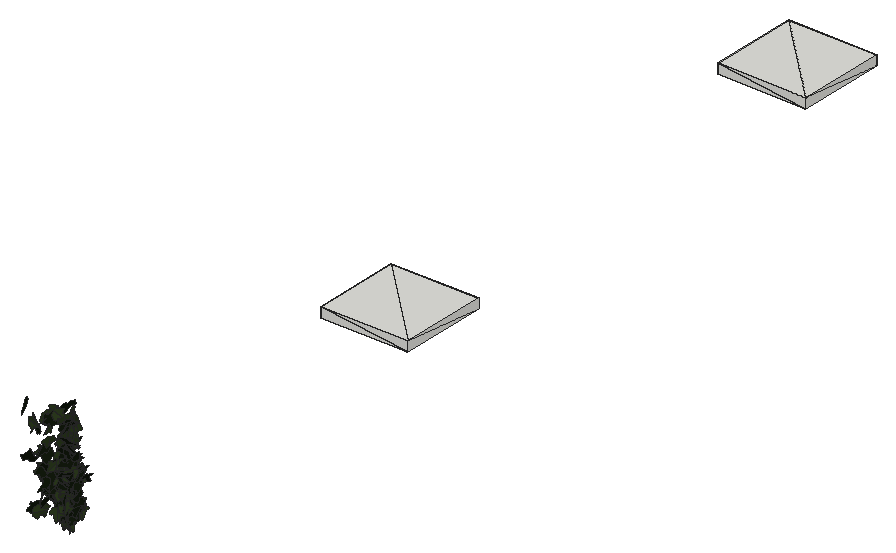
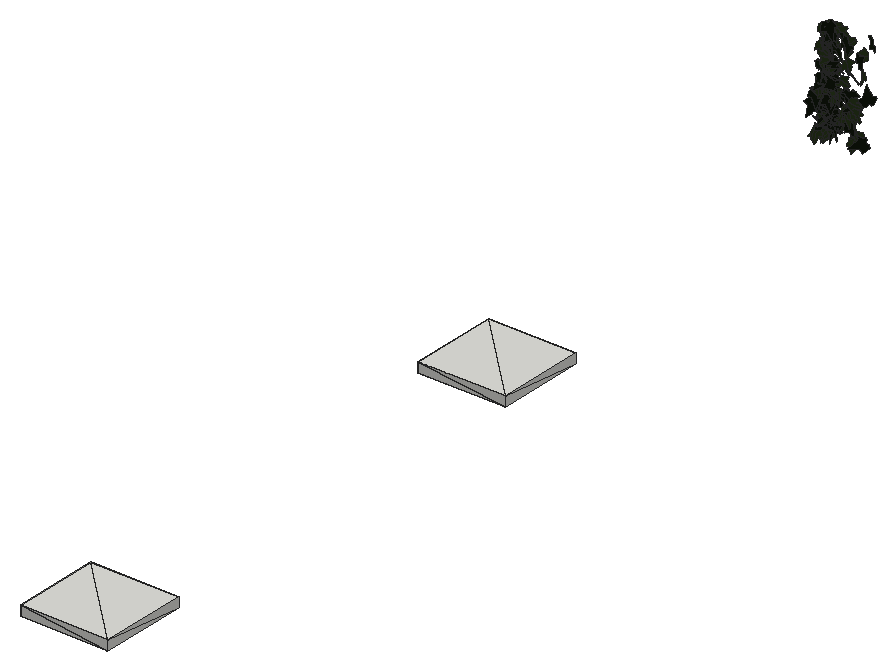
# SketchUp Ruby script. Lengths in inches.
U = 1.inch
M = Sketchup.active_model
def pt(a) = Geom::Point3d.new(a.map { |v| v * U })
def face(e, loops, mat)
  f = e.add_face(loops[0].map { |a| pt(a) })
  loops[1..].each { |l| e.add_face(l.map { |a| pt(a) }).erase! }
  f.material = f.back_material = mat if mat
  f
end
# faces: each face lists its corners as indices into pts; further lists are holes
def faces(e, pts, list, mat = nil) = list.each { |f| face(e, (f[0].is_a?(Array) ? f : [f]).map { |l| l.map { |i| pts[i] } }, mat) }
# xy, xz, yz: faces in a plane at the given z, y or x. An outline is a flat list of corners, or four numbers for a rectangle; further outlines are holes
def ring(l) = l.size == 4 ? [[l[0], l[1]], [l[2], l[1]], [l[2], l[3]], [l[0], l[3]]] : l.each_slice(2).to_a
def flat(e, list, mat, &to3) = list.each { |f| face(e, (f[0].is_a?(Array) ? f : [f]).map { |l| ring(l).map { |u, v| to3.(u, v) } }, mat) }
def xy(e, z, list, mat = nil) = flat(e, list, mat) { |x, y| [x, y, z] }
def xz(e, y, list, mat = nil) = flat(e, list, mat) { |x, z| [x, y, z] }
def yz(e, x, list, mat = nil) = flat(e, list, mat) { |y, z| [x, y, z] }
def lines(e, pts, list) = list.each { |a, b| e.add_line(pt(pts[a]), pt(pts[b])) }
# prism: a flat outline (further loops are holes) pulled along v
def prism(e, loops, v, mat = nil)
  f = face(e, loops, mat); d = Geom::Vector3d.new(v.map { |x| x * U })
  f.pushpull(f.normal.samedirection?(d) ? d.length : -d.length)
end
def box(e, o, s, mat = nil) = prism(e, [[o, [o[0] + s[0], o[1], o[2]], [o[0] + s[0], o[1] + s[1], o[2]], [o[0], o[1] + s[1], o[2]]]], [0, 0, s[2]], mat)
def at(x, y, z, deg = 0) = Geom::Transformation.translation(pt([x, y, z])) * Geom::Transformation.rotation(ORIGIN, Z_AXIS, deg.degrees)
def axes(o, x, y, z) = Geom::Transformation.new([*x, 0, *y, 0, *z, 0, *pt(o).to_a, 1])
def part(name) = M.definitions.add(name)
# library, detail: a bought-in or finely detailed component or shape, given as its bounding box
def library(name, o, s) = part(name).tap { |d| box(d.entities, o, s) }
def detail(e, o, s) = box(e.add_group.entities, o, s)
def put(e, d, t, mat = nil) = e.add_instance(d, t).tap { |i| i.material = mat if mat }
def group(e, t, mat = nil) = e.add_group.tap { |g| g.transformation = t; g.material = mat if mat }.entities
root = M.entities
M.materials.add("efeu1").color = [18, 25, 13]
M.materials.add("efeu2").color = [43, 57, 29]
c1 = part("ivyleaf_9")
p = [[1.54,2.16,1.25],[1.36,2.04,1.19],[-0.21,0.99,0.68],[-0.71,1.11,0.82],[-0.85,0.86,0.67],[-0.8,0.17,0.21],
  [-0.9,-0.01,0.1],[-0.67,-0.16,-0.02],[-0.08,-0.08,-0.05],[-0.03,-0.6,-0.4],[0.65,-0.88,-0.66],[0.83,-0.6,-0.49],
  [1.29,-0.42,-0.43],[1.8125,-0.07,-0.26],[1.21,0.44,0.15]]
faces(c1.entities,p,[[0,1,2,3,4,5,6,7,8,9,10,11,12,13,14]],"efeu1")
c2 = part("ivyleaf_10")
p = [[0,0.5,-0.03],[-0.0625,2.02,-0.43],[-0.19,2.01,-0.46],[-0.54,1.05,-0.29],[-0.52,0.625,-0.18],[-0.83,0.76,-0.28],
  [-1.16,0.64,-0.33],[-1.15,0.33,-0.24],[-0.77,-0.39,0.02],[-0.3,-0.51,0.16],[0.04,-0.48,0.23],[-0.02,2.01,-0.4375],
  [-0.06,2.01,-0.43],[0.04,-0.49,0.23],[0.67,-0.49,0.14],[1.38,0.36,-0.2],[1.375,0.51,-0.24],[0.81,0.65,-0.19],
  [0.62,0.59,-0.15],[0.6,1.09,-0.28],[0.5,1.23,-0.31]]
faces(c2.entities,p,[[0,1,2,3,4,5,6,7,8,9,10],[11,12,0,13,14,15,16,17,18,19,20]],"efeu2")
c3 = part("Tlon Cubo 860 Ceiling 152 005")
xy(c3.entities,-3.04,[[-16.54,-16.54,-16.54,16.54,16.54,-16.54],[16.54,-16.54,-16.54,16.54,16.54,16.54]])
xy(c3.entities,0,[[-16.93,-16.93,16.93,-16.93,-16.93,16.93],[16.93,-16.93,16.93,16.93,-16.93,16.93]])
xz(c3.entities,-16.93,[[-16.93,-3.79,16.93,-3.79,-16.93,0],[16.93,-3.79,16.93,0,-16.93,0]])
xz(c3.entities,-16.3,[[-16.3,-3.66,-16.3,-3.24,16.3,-3.24],[-16.3,-3.66,16.3,-3.24,16.3,-3.66]])
xz(c3.entities,16.3,[[-16.3,-3.66,16.3,-3.24,-16.3,-3.24],[-16.3,-3.66,16.3,-3.66,16.3,-3.24]])
xz(c3.entities,16.93,[[-16.93,-3.79,-16.93,0,16.93,0],[-16.93,-3.79,16.93,0,16.93,-3.79]])
yz(c3.entities,-16.93,[[-16.93,-3.79,-16.93,0,16.93,0],[-16.93,-3.79,16.93,0,16.93,-3.79]])
yz(c3.entities,-16.3,[[-16.3,-3.66,16.3,-3.66,-16.3,-3.24],[16.3,-3.66,16.3,-3.24,-16.3,-3.24]])
yz(c3.entities,16.3,[[-16.3,-3.66,-16.3,-3.24,16.3,-3.66],[16.3,-3.66,-16.3,-3.24,16.3,-3.24]])
yz(c3.entities,16.93,[[-16.93,-3.79,16.93,-3.79,-16.93,0],[16.93,-3.79,16.93,0,-16.93,0]])
p = [[-16.93,-16.93,-3.79],[-16.93,16.93,-3.79],[-16.3,16.3,-3.66],[-16.3,-16.3,-3.66],[16.93,-16.93,-3.79],[16.3,-16.3,-3.66],
  [16.93,16.93,-3.79],[16.3,16.3,-3.66]]
faces(c3.entities,p,[[0,1,2],[2,3,0],[4,0,3],[3,5,4],[6,4,5],[5,7,6],[2,1,6],[6,7,2]])
put(root,c1,axes([51.99,223.18,231.17],[-0.2698,0.42062,0.0171],[-0.00149,0.01936,-0.49962],[-0.42096,-0.26964,-0.0092]))
put(root,c1,axes([52.75,223.1875,232.52],[-0.29908,0.34224,0.20838],[-0.15446,0.14146,-0.45402],[-0.36972,-0.33595,0.02111]))
put(root,c2,axes([51.98,223.04,231.11],[-0.05835,-0.15634,-0.47133],[0.27915,0.38216,-0.16132],[0.41069,-0.28197,0.04269]))
put(root,c2,axes([51.42,223.35,224.12],[0.49188,0.07377,0.05109],[0.04249,0.05928,-0.49465],[-0.07903,0.49096,0.05205]))
put(root,c2,axes([51.83,223.35,227.09],[0.41897,0.26721,0.05532],[0.04014,0.0399,-0.49679],[-0.26991,0.42072,0.01198]))
put(root,c2,axes([51.9,223.12,226.03],[0.14823,0.31759,0.3566],[0.16019,0.31868,-0.35041],[-0.44985,0.21813,-0.00727]))
put(root,c2,axes([51.17,223.53,228.35],[0.25617,0.2671,-0.33621],[-0.2769,-0.19647,-0.36705],[-0.32819,0.37425,0.04726]))
put(root,c2,axes([49.46,223.08,223.48],[-0.01779,0.00376,-0.49967],[0.37702,0.32823,-0.01096],[0.32793,-0.37716,-0.01452]))
put(root,c2,axes([52.16,223.51,223.72],[0.4327,-0.1789,0.1754],[0.15861,-0.07536,-0.46815],[0.19394,0.46078,-0.00847]))
put(root,c1,axes([52.6875,223.53,229.21],[-0.48442,0.0135,0.1231],[-0.12323,-0.00334,-0.48457],[-0.01226,-0.49981,0.00656]))
put(root,c2,axes([52.29,223.27,233.11],[-0.25276,-0.36738,-0.22616],[0.125,0.1885,-0.44592],[0.4129,-0.28196,-0.00344]))
put(root,c1,axes([51.8125,223.5625,226.1],[-0.20105,-0.12133,-0.44143],[0.44485,0.0621,-0.21967],[0.10813,-0.48106,0.08298]))
put(root,c1,axes([52.4375,223.21,232.44],[-0.12321,0.28045,0.39518],[-0.31389,0.26446,-0.28554],[-0.36918,-0.31845,0.11089]))
put(root,c1,axes([52.09,223.28,230.91],[0.38814,-0.08975,0.30215],[0.31308,0.05435,-0.38604],[0.03645,0.48887,0.09839]))
put(root,c1,axes([50.71,223.29,232.12],[-0.35338,0.16607,0.31232],[0.28365,-0.13074,0.39045],[0.21135,0.45313,-0.00181]))
put(root,c1,axes([48.23,223.05,232.59],[0.008,0.18928,0.46272],[-0.04717,0.461,-0.18776],[-0.49771,-0.04064,0.02524]))
put(root,c2,axes([48.65,223.4375,231.43],[0.06141,-0.02418,0.49563],[0.49265,0.06273,-0.05798],[-0.05937,0.49546,0.03153]))
put(root,c2,axes([52.33,223.42,231.79],[-0.21445,-0.44743,-0.06176],[0.04201,0.04832,-0.49588],[0.44972,-0.21787,0.01687]))
put(root,c2,axes([51.67,223.52,229.37],[0.25967,0.40462,-0.13731],[-0.0643,-0.12184,-0.48065],[-0.42242,0.26727,-0.01124]))
put(root,c2,axes([52.83,223.2,223.25],[-0.15601,0.20068,0.43057],[-0.37656,0.22403,-0.24086],[-0.28959,-0.39942,0.08123]))
put(root,c1,axes([51.99,223.33,226.23],[-0.09202,-0.05056,0.48885],[0.49146,-0.01021,0.09146],[0.00073,0.49733,0.05158]))
put(root,c1,axes([52.02,223.53,229.86],[-0.47148,0.1548,-0.06123],[0.05447,-0.03033,-0.4961],[-0.1573,-0.47447,0.01174]))
put(root,c1,axes([50.14,223.32,225.52],[0.49981,0.01188,0.007],[0.00686,0.00583,-0.49992],[-0.01196,0.49982,0.00566]))
put(root,c1,axes([51.68,223.66,226.14],[-0.43269,-0.03139,0.24858],[-0.24779,-0.01994,-0.43383],[0.03715,-0.49861,0.0017]))
put(root,c2,axes([52.15,223.27,226.09],[-0.17913,-0.21497,-0.41436],[0.29934,0.28766,-0.27865],[0.3582,-0.34791,0.02564]))
put(root,c1,axes([52.22,223.69,226.79],[-0.21053,-0.45189,-0.03835],[0.00457,-0.04439,0.498],[-0.45349,0.20934,0.02282]))
put(root,c2,axes([52.26,223.37,224.43],[0.25577,0.40736,-0.13652],[0.07693,0.11289,0.48097],[0.42268,-0.26705,-0.00493]))
put(root,c1,axes([52.28,223.6,232.37],[-0.29082,0.31838,-0.2531],[0.17374,-0.18408,-0.43119],[-0.36775,-0.33874,-0.00356]))
put(root,c1,axes([51.2,223.76,227.13],[-0.43377,-0.23411,-0.08387],[0.07428,0.03895,-0.49291],[0.23733,-0.44008,0.00099]))
put(root,c1,axes([52,223.66,225.13],[-0.14139,-0.43178,-0.20873],[0.07281,0.19577,-0.45428],[0.47403,-0.15886,0.00752]))
put(root,c1,axes([51.74,223.5,229.55],[0.33446,0.10812,-0.3556],[0.30194,0.19992,0.34477],[0.21673,-0.44536,0.06844]))
put(root,c1,axes([52.15,223.41,224.18],[-0.15793,0.01591,-0.47414],[-0.4744,-0.00795,0.15775],[-0.00252,0.49968,0.01761]))
put(root,c1,axes([52.38,223.33,232.76],[0.38647,0.31304,-0.05145],[-0.04028,-0.032,-0.49735],[-0.31467,0.38857,0.00049]))
put(root,c2,axes([51.79,223.66,226.875],[0.44058,-0.11145,0.20849],[0.20667,-0.03253,-0.45412],[0.11479,0.48633,0.0174]))
put(root,c2,axes([51.67,223.54,226.35],[-0.16276,0.46935,-0.05673],[0.02778,-0.0504,-0.49668],[-0.47195,-0.16483,-0.00967]))
put(root,c2,axes([51.33,223.4,233.17],[0.20313,0.22085,0.39995],[0.27389,0.29147,-0.30005],[-0.36568,0.34099,-0.00256]))
put(root,c2,axes([50.27,223.93,231.39],[-0.0838,0.22244,-0.43988],[-0.08532,-0.446,-0.20928],[-0.48549,0.03999,0.11271]))
put(root,c1,axes([52.66,223.8,229.11],[0.25266,0.0815,0.4237],[-0.40549,-0.12294,0.26545],[0.14745,-0.47775,0.00397]))
put(root,c1,axes([52.27,223.44,227.79],[0.24133,0.40949,-0.15517],[-0.11368,-0.11252,-0.47373],[-0.42289,0.26393,0.03879]))
put(root,c1,axes([52.16,223.47,223.72],[0.33089,0.0139,-0.37459],[-0.37485,0.01358,-0.33061],[0.00098,0.49962,0.01941]))
put(root,c1,axes([50.21,224.05,225.88],[-0.22521,-0.28219,0.3459],[-0.1465,-0.31925,-0.35583],[0.42169,-0.26162,0.06112]))
put(root,c2,axes([50.4,223.73,230.3],[-0.15151,-0.47289,0.05849],[-0.02423,-0.05365,-0.49652],[0.47587,-0.1533,-0.00666]))
put(root,c2,axes([52.02,223.68,229.14],[0.43207,0.25151,0.00775],[0.00663,0.00401,-0.49994],[-0.25154,0.43212,0.00014]))
put(root,c1,axes([51.65,223.92,224.62],[0.16405,-0.45201,0.13701],[0.0572,-0.12496,-0.48074],[0.46885,0.1734,0.01071]))
put(root,c1,axes([50.16,223.69,224.71],[-0.15401,0.41811,-0.22687],[0.08045,-0.21213,-0.44556],[-0.46884,-0.17374,-0.00194]))
put(root,c2,axes([52.0625,223.63,229.79],[-0.2564,0.42896,-0.01595],[0.01032,-0.01241,-0.49974],[-0.42913,-0.2566,-0.00249]))
put(root,c1,axes([50.1,223.8,229.64],[-0.4738,0.12838,-0.09505],[0.09137,-0.02622,-0.49088],[-0.13102,-0.48253,0.00138]))
put(root,c2,axes([52.75,223.86,228.17],[0.24115,0.12742,-0.41906],[-0.39484,-0.14384,-0.27094],[-0.1896,0.4616,0.03125]))
put(root,c2,axes([52.36,223.74,232.29],[0.46314,-0.13571,-0.13072],[-0.11582,0.06859,-0.48154],[0.14863,0.47632,0.03209]))
put(root,c2,axes([51.99,223.7,228.59],[-0.06423,-0.48765,-0.08985],[0.01804,0.08824,-0.49182],[0.49553,-0.06642,0.00626]))
put(root,c2,axes([49.99,223.38,232.25],[-0.00602,0.16139,0.4732],[0.02084,0.4729,-0.16102],[-0.49953,0.01778,-0.01242]))
put(root,c1,axes([52.72,223.42,227.49],[-0.01797,0.19822,0.45868],[-0.12759,0.44194,-0.19598],[-0.48311,-0.12409,0.0347]))
put(root,c1,axes([51.875,223.76,223.65],[-0.43716,-0.20329,-0.13253],[-0.12019,-0.05585,0.48212],[-0.21083,0.45338,-0.00003]))
put(root,c2,axes([51,223.81,233.2],[0.29772,0.07491,-0.39465],[-0.3993,0.00155,-0.30093],[-0.04386,0.49435,0.06074]))
put(root,c1,axes([52.11,223.48,224.37],[0.00078,-0.07456,0.49441],[0.04896,0.49205,0.07413],[-0.4976,0.04829,0.00807]))
put(root,c1,axes([52.37,223.68,230.3],[0.48035,-0.0238,-0.13673],[-0.13657,0.00667,-0.48094],[0.02472,0.49939,-0.00009]))
put(root,c1,axes([47.95,223.93,227.53],[0.44818,0.16239,0.15087],[-0.14222,-0.05036,0.47669],[0.17002,-0.4702,0.00105]))
put(root,c2,axes([49.29,223.85,223.92],[0.30684,-0.39426,0.0202],[-0.01169,0.0165,0.49959],[-0.3946,-0.30706,0.00091]))
put(root,c1,axes([49.17,223.72,230.67],[0.08728,-0.15157,0.46841],[-0.20756,0.42004,0.17459],[-0.44643,-0.22492,0.0104]))
put(root,c1,axes([51.63,223.86,226.86],[0.43358,-0.2296,0.09643],[0.08619,-0.04329,-0.49061],[0.23363,0.44205,0.00204]))
put(root,c1,axes([52.7,223.9,223.47],[-0.36283,-0.33132,0.09264],[0.07111,0.0595,0.49133],[-0.3366,0.36971,0.00395]))
put(root,c2,axes([52.15,223.71,223.17],[0.18415,0.3888,0.25481],[0.10964,0.23001,-0.4302],[-0.45174,0.21432,-0.00054]))
put(root,c1,axes([51.79,223.82,224.85],[-0.00019,-0.30182,-0.39863],[0.07241,0.39441,-0.29866],[0.49473,-0.05784,0.04356]))
put(root,c1,axes([51.56,223.65,223.17],[0.08431,-0.04831,0.49047],[-0.02416,0.49659,0.05306],[-0.49225,-0.03265,0.0814]))
put(root,c1,axes([50.0625,223.79,227.7],[0.34887,0.25709,-0.24939],[-0.1999,-0.14913,-0.43336],[-0.29721,0.40208,-0.00127]))
put(root,c1,axes([52.3,223.79,223.62],[-0.16732,-0.00407,0.47116],[0.47091,0.01521,0.16736],[-0.0157,0.49975,-0.00126]))
put(root,c2,axes([50.43,224.31,225.8],[-0.05732,0.11531,0.48313],[0.17058,-0.45219,0.12816],[0.46649,0.17952,0.0125]))
put(root,c1,axes([48.57,223.65,223.43],[0.07198,0.15473,-0.46998],[0.11238,0.4574,0.1678],[0.48186,-0.12979,0.03107]))
put(root,c2,axes([50.26,224.06,225.43],[0.45716,-0.16851,-0.11227],[-0.10149,0.04919,-0.48711],[0.17522,0.46817,0.01077]))
put(root,c1,axes([52.43,223.94,231.65],[-0.31838,0.38098,0.05908],[-0.03657,0.04643,-0.49649],[-0.38379,-0.32047,-0.0017]))
put(root,c2,axes([50.33,223.96,225.14],[0.09879,0.02192,0.48965],[0.45419,0.18367,-0.09985],[-0.18425,0.46452,0.01638]))
put(root,c1,axes([52.1875,224.37,228.5],[-0.41413,-0.25718,0.11116],[-0.0944,-0.0587,-0.48749],[0.2638,-0.42475,0.00006]))
put(root,c2,axes([49.41,224.06,223.45],[-0.26554,-0.41015,-0.10613],[0.07905,0.07508,-0.48797],[0.41622,-0.27593,0.02497]))
put(root,c1,axes([50.19,223.8125,232.42],[-0.07002,0.44725,0.21229],[-0.0152,0.21236,-0.45241],[-0.49484,-0.0698,-0.01614]))
put(root,c1,axes([51.68,224.45,230.05],[-0.38252,-0.29209,0.13551],[-0.1018,-0.08992,-0.4812],[0.30548,-0.39572,0.00933]))
put(root,c1,axes([52.34,223.84,223.4],[0.08078,0.04507,0.49137],[0.37939,0.31268,-0.09105],[-0.31549,0.38755,0.01632]))
put(root,c1,axes([50.38,223.77,232.6],[0.09696,0.34198,0.35163],[-0.01452,0.36028,-0.34639],[-0.49029,0.05696,0.07979]))
put(root,c1,axes([51.8,223.79,232.7],[0.16563,0.34897,0.31747],[0.03912,0.32515,-0.37782],[-0.47015,0.14999,0.08041]))
put(root,c2,axes([52.65,224.14,231.62],[0.01211,0.0473,0.49761],[-0.49831,0.04018,0.0083],[-0.03921,-0.49613,0.04812]))
put(root,c2,axes([52.25,223.88,223.32],[0.03382,-0.05755,0.49552],[0.04088,0.49531,0.05473],[-0.49718,0.03681,0.03821]))
put(root,c1,axes([52.71,224.47,226.67],[-0.47375,-0.08482,0.13552],[-0.13233,-0.02979,-0.48125],[0.08971,-0.49185,0.00578]))
put(root,c2,axes([52.68,224.27,230.99],[-0.08201,0.01492,0.493],[-0.48867,-0.07022,-0.07916],[0.06688,-0.49482,0.0261]))
put(root,c2,axes([50.48,224.19,225.64],[-0.1664,0.46707,0.06449],[-0.02822,0.0584,-0.49578],[-0.47065,-0.16864,0.00692]))
put(root,c2,axes([52.68,224.1875,233.15],[-0.37153,0.20119,0.26736],[-0.25662,0.08505,-0.42061],[-0.21473,-0.44976,0.04006]))
put(root,c2,axes([50.58,224.42,227.33],[-0.28428,0.33512,-0.23849],[0.11145,-0.2163,-0.4368],[-0.39593,-0.30151,0.04828]))
put(root,c1,axes([52.29,224.54,227.72],[-0.25336,0.12418,-0.41278],[0.36884,-0.18534,-0.28215],[-0.22309,-0.44747,0.00231]))
put(root,c1,axes([49.28,224.55,226.74],[-0.21665,-0.42012,-0.16297],[0.12048,0.12024,-0.47013],[0.43422,-0.24298,0.04914]))
put(root,c2,axes([52.56,224.46,231.8125],[0.04089,0.47772,-0.14181],[-0.17135,-0.12013,-0.4541],[-0.46794,0.08573,0.15389]))
put(root,c2,axes([52.11,224.11,228.4375],[-0.00423,-0.08233,0.49316],[0.14275,0.47245,0.0801],[-0.47917,0.14148,0.01951]))
put(root,c1,axes([51.77,224.375,233.76],[0.01258,0.45493,-0.20708],[-0.02359,-0.20638,-0.45481],[-0.49929,0.02121,0.01627]))
put(root,c2,axes([51.68,224.45,228.26],[-0.0692,0.49334,-0.04269],[0.001,-0.04296,-0.49815],[-0.49519,-0.06903,0.00496]))
put(root,c2,axes([48.96,224.6,226.49],[-0.3744,-0.32315,0.07351],[-0.02174,-0.08673,-0.49194],[0.33069,-0.37156,0.05089]))
put(root,c1,axes([51.98,224.74,225.98],[-0.46552,-0.12768,-0.13035],[0.1294,0.02079,-0.48252],[0.12863,-0.48298,0.01369]))
put(root,c1,axes([49.32,224.71,228.41],[-0.30465,-0.31205,-0.24457],[0.19255,0.15317,-0.43528],[0.34658,-0.35939,0.02684]))
put(root,c2,axes([52.17,224.4,223.65],[0.01361,0.47364,0.15962],[-0.02892,0.16016,-0.47277],[-0.49898,0.00364,0.03175]))
put(root,c1,axes([52.26,224.4,226.29],[0.25996,-0.07481,-0.42051],[-0.37706,0.19102,-0.26709],[0.20061,0.45598,0.0429]))
put(root,c1,axes([52.95,224.53,224.55],[-0.32444,0.27647,0.26134],[-0.22473,0.13787,-0.42484],[-0.30697,-0.39314,0.0348]))
put(root,c1,axes([51.74,224.52,228.83],[-0.11987,0.2067,0.43921],[-0.40127,0.21238,-0.20947],[-0.27315,-0.40271,0.11497]))
put(root,c2,axes([52.28,224.46,229.42],[-0.28183,0.34859,0.22149],[-0.16779,0.14838,-0.44702],[-0.37739,-0.3263,0.03335]))
put(root,c1,axes([52.375,224.62,226.48],[-0.01716,0.41804,-0.27376],[-0.0685,-0.27331,-0.41305],[-0.49499,0.02333,0.06665]))
put(root,c2,axes([52.14,224.43,233.06],[-0.2313,0.34607,0.27702],[-0.14961,0.23319,-0.41622],[-0.41728,-0.27543,-0.00432]))
put(root,c2,axes([50.98,224.51,227.17],[-0.04798,0.47791,0.13892],[-0.00063,0.13951,-0.48014],[-0.49769,-0.04625,-0.01278]))
put(root,c2,axes([51.77,224.48,230.28],[0.21707,0.1625,0.42009],[0.3003,0.29535,-0.26942],[-0.33571,0.36927,0.03062]))
put(root,c1,axes([52.23,225.05,227.95],[-0.24243,-0.43721,0.00877],[0.08341,-0.05608,-0.48979],[0.42927,-0.23602,0.10012]))
put(root,c1,axes([50.95,224.65,228.66],[0.34456,0.33488,-0.13832],[0.0927,0.10306,0.4804],[0.35027,-0.3567,0.00893]))
put(root,c2,axes([48.05,224.52,230.43],[0.06195,-0.28871,-0.4035],[-0.074,0.39671,-0.29521],[0.4906,0.09629,0.00642]))
put(root,c1,axes([52.76,224.6,227.16],[-0.2015,0.35821,0.28475],[-0.23494,0.18601,-0.40025],[-0.39268,-0.2951,0.09336]))
put(root,c1,axes([52.25,225.04,228.07],[-0.44988,-0.08253,0.20199],[-0.19182,-0.07102,-0.45625],[0.104,-0.488,0.03224]))
put(root,c1,axes([52.6,224.65,225.26],[-0.14219,0.18803,0.44094],[-0.31291,0.31201,-0.23396],[-0.36314,-0.34248,0.02894]))
put(root,c1,axes([51.93,224.59,225.94],[0.27538,0.41639,0.02797],[0.01376,0.02443,-0.49921],[-0.4171,0.27572,0.00199]))
put(root,c1,axes([51.36,224.7,227.0625],[0.07066,0.48513,-0.09828],[-0.01534,-0.09708,-0.49024],[-0.49474,0.07229,0.00116]))
put(root,c2,axes([51,224.54,227.41],[0.07989,0.20363,0.44961],[-0.30211,0.38035,-0.11858],[-0.39032,-0.25272,0.18381]))
put(root,c2,axes([48.87,224.82,226.65],[0.31166,0.06218,-0.38601],[-0.38214,0.15285,-0.28391],[0.0827,0.47198,0.1428]))
put(root,c1,axes([52.38,224.86,230.07],[-0.30572,0.39539,0.0142],[-0.00728,0.01232,-0.4998],[-0.39558,-0.3058,-0.00178]))
put(root,c2,axes([52.32,225.13,226.87],[0.24489,0.36004,-0.24576],[-0.13481,-0.20552,-0.43542],[-0.41455,0.27952,-0.00359]))
put(root,c2,axes([52.35,225.03,227.71],[-0.3806,-0.32232,0.03539],[-0.01049,-0.0423,-0.4981],[0.32409,-0.37989,0.02543]))
put(root,c1,axes([51.88,224.68,228.8],[0.37275,0.30534,0.1335],[0.01404,0.18573,-0.46401],[-0.33296,0.34967,0.12988]))
put(root,c2,axes([51.83,224.83,225.38],[0.11825,0.32711,0.35919],[-0.00305,0.37017,-0.3361],[-0.48581,0.07729,0.08954]))
put(root,c1,axes([52.31,225.15,226.23],[-0.38736,0.3087,-0.06824],[0.04623,-0.05146,-0.49519],[-0.31275,-0.38995,0.01132]))
put(root,c2,axes([48.65,225.29,227.91],[0.21533,0.03483,-0.44991],[-0.44511,-0.0656,-0.21811],[-0.07422,0.49445,0.00276]))
put(root,c1,axes([52.49,225.14,227.4375],[-0.00914,0.49902,0.02989],[0.00285,0.02995,-0.49909],[-0.49991,-0.00895,-0.00339]))
put(root,c2,axes([52.29,225.32,223.8],[0.22448,0.43925,0.08167],[0.0056,0.08862,-0.49205],[-0.44674,0.22182,0.03487]))
put(root,c2,axes([52.45,225.46,224.4],[-0.23388,0.43001,0.10192],[-0.05657,0.08523,-0.48942],[-0.43829,-0.24047,0.00879]))
put(root,c1,axes([52.5,225.35,226.63],[0.19331,0.43683,0.14767],[0.05908,0.13533,-0.4777],[-0.45732,0.20214,0.0007]))
put(root,c3,axes([50.28,269.25,222.96],[0.2697,0,0],[0,0.2697,0],[0,0,0.2697]))
put(root,c3,axes([50.28,320.87,222.96],[0.2697,0,0],[0,0.2697,0],[0,0,0.2697]))
